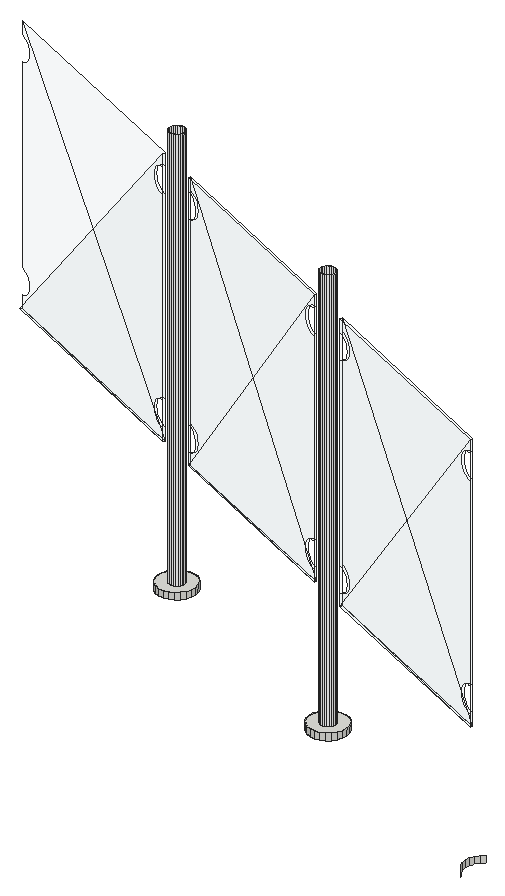
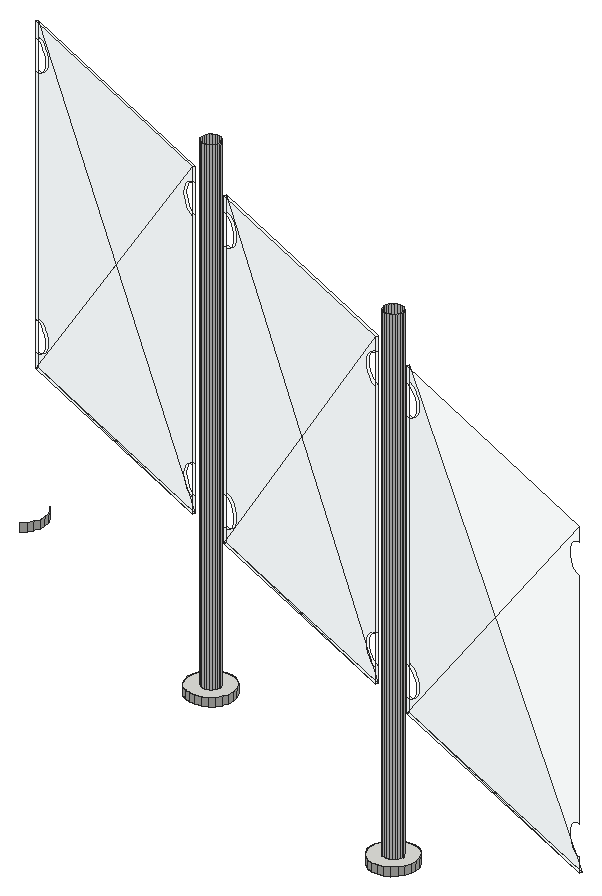
# SketchUp Ruby script. Lengths in inches.
U = 1.inch
M = Sketchup.active_model
def pt(a) = Geom::Point3d.new(a.map { |v| v * U })
def face(e, loops, mat)
  f = e.add_face(loops[0].map { |a| pt(a) })
  loops[1..].each { |l| e.add_face(l.map { |a| pt(a) }).erase! }
  f.material = f.back_material = mat if mat
  f
end
# faces: each face lists its corners as indices into pts; further lists are holes
def faces(e, pts, list, mat = nil) = list.each { |f| face(e, (f[0].is_a?(Array) ? f : [f]).map { |l| l.map { |i| pts[i] } }, mat) }
# xy, xz, yz: faces in a plane at the given z, y or x. An outline is a flat list of corners, or four numbers for a rectangle; further outlines are holes
def ring(l) = l.size == 4 ? [[l[0], l[1]], [l[2], l[1]], [l[2], l[3]], [l[0], l[3]]] : l.each_slice(2).to_a
def flat(e, list, mat, &to3) = list.each { |f| face(e, (f[0].is_a?(Array) ? f : [f]).map { |l| ring(l).map { |u, v| to3.(u, v) } }, mat) }
def xy(e, z, list, mat = nil) = flat(e, list, mat) { |x, y| [x, y, z] }
def xz(e, y, list, mat = nil) = flat(e, list, mat) { |x, z| [x, y, z] }
def yz(e, x, list, mat = nil) = flat(e, list, mat) { |y, z| [x, y, z] }
def lines(e, pts, list) = list.each { |a, b| e.add_line(pt(pts[a]), pt(pts[b])) }
# prism: a flat outline (further loops are holes) pulled along v
def prism(e, loops, v, mat = nil)
  f = face(e, loops, mat); d = Geom::Vector3d.new(v.map { |x| x * U })
  f.pushpull(f.normal.samedirection?(d) ? d.length : -d.length)
end
def box(e, o, s, mat = nil) = prism(e, [[o, [o[0] + s[0], o[1], o[2]], [o[0] + s[0], o[1] + s[1], o[2]], [o[0], o[1] + s[1], o[2]]]], [0, 0, s[2]], mat)
def at(x, y, z, deg = 0) = Geom::Transformation.translation(pt([x, y, z])) * Geom::Transformation.rotation(ORIGIN, Z_AXIS, deg.degrees)
def axes(o, x, y, z) = Geom::Transformation.new([*x, 0, *y, 0, *z, 0, *pt(o).to_a, 1])
def part(name) = M.definitions.add(name)
# library, detail: a bought-in or finely detailed component or shape, given as its bounding box
def library(name, o, s) = part(name).tap { |d| box(d.entities, o, s) }
def detail(e, o, s) = box(e.add_group.entities, o, s)
def put(e, d, t, mat = nil) = e.add_instance(d, t).tap { |i| i.material = mat if mat }
def group(e, t, mat = nil) = e.add_group.tap { |g| g.transformation = t; g.material = mat if mat }.entities
root = M.entities
M.materials.add("Glass_Safety_01").color = [204, 235, 244]
M.materials["Glass_Safety_01"].alpha = 0.1
M.materials.add("[Color_000]").color = [255, 255, 255]
xy(root,321.27,[[[766.1875,566.06,766.59,566.14,766.96,566.32,767.27,566.6,767.49,566.94,767.62,567.33,767.65,567.74,767.5625,568.14,767.38,568.51,767.11,568.82,766.76,569.04,766.375,569.17,765.96,569.2,765.5625,569.12,765.19,568.93,764.89,568.66,764.66,568.32,764.64,568.25,764.53,567.93,764.51,567.52,764.59,567.11,764.77,566.75,765.05,566.4375,765.39,566.21,765.78,566.08],[766.12,567,765.96,567.01,765.8,567.0625,765.66,567.15,765.55,567.28,765.48,567.42,765.45,567.58,765.46,567.75,765.5,567.88,765.51,567.9,765.6,568.04,765.72,568.15,765.87,568.22,766.03,568.26,766.2,568.25,766.35,568.19,766.49,568.1,766.6,567.98,766.67,567.83,766.7,567.67,766.69,567.51,766.65,567.38,766.64,567.35,766.55,567.22,766.43,567.11,766.28,567.03]],[767.51,567,767.62,567.33,767.65,567.74,767.5625,568.14,767.38,568.51,767.11,568.82,766.76,569.04,766.375,569.17,765.96,569.2,765.5625,569.12,765.19,568.93,764.89,568.66,764.66,568.32,764.64,568.25,765.5,567.88,765.51,567.9,765.6,568.04,765.72,568.15,765.87,568.22,766.03,568.26,766.2,568.25,766.35,568.19,766.49,568.1,766.6,567.98,766.67,567.83,766.7,567.67,766.69,567.51,766.65,567.38],[766.65,567.38,766.69,567.51,766.7,567.67,766.67,567.83,766.6,567.98,766.49,568.1,766.35,568.19,766.2,568.25,766.03,568.26,765.87,568.22,765.72,568.15,765.6,568.04,765.51,567.9,765.5,567.88],[[745.84,574.92,746.25,575,746.61,575.1875,746.92,575.46,747.15,575.8,747.28,576.19,747.3,576.6,747.22,577,747.03,577.37,746.76,577.68,746.42,577.91,746.03,578.04,745.62,578.06,745.21,577.98,744.85,577.79,744.54,577.52,744.3125,577.18,744.29,577.12,744.18,576.79,744.16,576.38,744.24,575.97,744.43,575.61,744.7,575.3,745.04,575.07,745.43,574.94],[745.78,575.86,745.61,575.87,745.45,575.92,745.32,576.01,745.21,576.14,745.13,576.28,745.1,576.44,745.11,576.61,745.16,576.74,745.16,576.76,745.25,576.9,745.375,577.01,745.52,577.08,745.68,577.12,745.85,577.11,746.01,577.06,746.14,576.97,746.25,576.84,746.33,576.7,746.36,576.53,746.35,576.37,746.3,576.24,746.3,576.21,746.21,576.08,746.08,575.97,745.9375,575.89]],[747.17,575.86,747.28,576.19,747.3,576.6,747.22,577,747.03,577.37,746.76,577.68,746.42,577.91,746.03,578.04,745.62,578.06,745.21,577.98,744.85,577.79,744.54,577.52,744.3125,577.18,744.29,577.12,745.16,576.74,745.16,576.76,745.25,576.9,745.375,577.01,745.52,577.08,745.68,577.12,745.85,577.11,746.01,577.06,746.14,576.97,746.25,576.84,746.33,576.7,746.36,576.53,746.35,576.37,746.3,576.24],
  [746.3,576.24,746.35,576.37,746.36,576.53,746.33,576.7,746.25,576.84,746.14,576.97,746.01,577.06,745.85,577.11,745.68,577.12,745.52,577.08,745.375,577.01,745.25,576.9,745.16,576.76,745.16,576.74]])
xy(root,321.27,[[766.12,567,766.28,567.03,766.43,567.11,766.55,567.22,766.64,567.35,766.65,567.38,765.5,567.88,765.46,567.75,765.45,567.58,765.48,567.42,765.55,567.28,765.66,567.15,765.8,567.0625,765.96,567.01],[745.78,575.86,745.9375,575.89,746.08,575.97,746.21,576.08,746.3,576.21,746.3,576.24,745.16,576.74,745.11,576.61,745.1,576.44,745.13,576.28,745.21,576.14,745.32,576.01,745.45,575.92,745.61,575.87]],"[Color_000]")
xy(root,321.86,[[766.1875,566.06,766.59,566.14,766.96,566.32,767.27,566.6,767.49,566.94,767.62,567.33,767.65,567.74,767.5625,568.14,767.38,568.51,767.11,568.82,766.76,569.04,766.375,569.17,765.96,569.2,765.5625,569.12,765.19,568.93,764.89,568.66,764.66,568.32,764.53,567.93,764.51,567.52,764.59,567.11,764.77,566.75,765.05,566.4375,765.39,566.21,765.78,566.08],[745.84,574.92,746.25,575,746.61,575.1875,746.92,575.46,747.15,575.8,747.28,576.19,747.3,576.6,747.22,577,747.03,577.37,746.76,577.68,746.42,577.91,746.03,578.04,745.62,578.06,745.21,577.98,744.85,577.79,744.54,577.52,744.3125,577.18,744.18,576.79,744.16,576.38,744.24,575.97,744.43,575.61,744.7,575.3,745.04,575.07,745.43,574.94]])
xy(root,331.9,[[785.36,559.12,767.84,566.75,767.92,566.93],[785.36,559.12,767.92,566.93,785.44,559.3],[764.39,568.25,747.5,575.61,747.57,575.79],[764.39,568.25,747.57,575.79,764.47,568.43],[744.03,577.12,724.79,585.5,724.87,585.68],
  [744.03,577.12,724.87,585.68,744.11,577.3]],"Glass_Safety_01")
p = [[785.75,557.61,321.27],[786.02,557.3,321.27],[786.02,557.3,321.86],[785.75,557.61,321.86],[785.5625,557.98,321.27],[785.5625,557.98,321.86],
  [785.48,558.38,321.27],[785.48,558.38,321.86],[785.51,558.79,321.27],[785.51,558.79,321.86],[785.64,559.18,321.27],[785.62,559.12,321.27],
  [785.64,559.18,321.86],[785.86,559.52,321.27],[785.86,559.52,321.86],[786.17,559.8,321.27],[786.17,559.8,321.86],[765.39,566.21,321.27],
  [765.78,566.08,321.27],[765.78,566.08,321.86],[765.39,566.21,321.86],[766.1875,566.06,321.27],[766.1875,566.06,321.86],[766.59,566.14,321.27],
  [766.59,566.14,321.86],[766.96,566.32,321.27],[766.96,566.32,321.86],[765.05,566.4375,321.27],[765.05,566.4375,321.86],[767.27,566.6,321.27],
  [767.27,566.6,321.86],[764.77,566.75,321.27],[764.77,566.75,321.86],[767.49,566.94,321.27],[767.49,566.94,321.86],[764.59,567.11,321.27],
  [764.59,567.11,321.86],[767.51,567,321.27],[767.62,567.33,321.27],[767.62,567.33,321.86],[765.8,567.0625,321.27],[765.96,567.01,321.27],
  [765.96,567.01,357.27],[765.8,567.0625,357.27],[766.12,567,321.27],[766.12,567,357.27],[766.28,567.03,321.27],[766.28,567.03,357.27],
  [766.43,567.11,321.27],[766.43,567.11,357.27],[764.51,567.52,321.27],[764.51,567.52,321.86],[765.66,567.15,321.27],[765.66,567.15,357.27],
  [766.55,567.22,321.27],[766.55,567.22,357.27],[765.55,567.28,321.27],[765.55,567.28,357.27],[766.64,567.35,321.27],[766.64,567.35,357.27],
  [765.48,567.42,321.27],[765.48,567.42,357.27],[767.65,567.74,321.27],[767.65,567.74,321.86],[765.45,567.58,321.27],[765.45,567.58,357.27],
  [766.65,567.38,321.27],[766.69,567.51,321.27],[766.69,567.51,357.27],[764.53,567.93,321.27],[764.53,567.93,321.86],[766.7,567.67,321.27],
  [766.7,567.67,357.27],[765.46,567.75,321.27],[765.46,567.75,357.27],[765.51,567.9,321.27],[765.5,567.88,321.27],[765.51,567.9,357.27],
  [766.67,567.83,321.27],[766.67,567.83,357.27],[767.5625,568.14,321.27],[767.5625,568.14,321.86],[766.6,567.98,321.27],[766.6,567.98,357.27],
  [764.66,568.32,321.27],[764.64,568.25,321.27],[764.66,568.32,321.86],[765.6,568.04,321.27],[765.6,568.04,357.27],[765.72,568.15,321.27],
  [765.72,568.15,357.27],[766.49,568.1,321.27],[766.49,568.1,357.27],[765.87,568.22,321.27],[765.87,568.22,357.27],[766.35,568.19,321.27],
  [766.35,568.19,357.27],[767.38,568.51,321.27],[767.38,568.51,321.86],[766.03,568.26,321.27],[766.03,568.26,357.27],[766.2,568.25,321.27],
  [766.2,568.25,357.27],[764.89,568.66,321.27],[764.89,568.66,321.86],[767.11,568.82,321.27],[767.11,568.82,321.86],[765.19,568.93,321.27],
  [765.19,568.93,321.86],[766.76,569.04,321.27],[766.76,569.04,321.86],[765.5625,569.12,321.27],[765.5625,569.12,321.86],[766.375,569.17,321.27],
  [766.375,569.17,321.86],[765.96,569.2,321.27],[765.96,569.2,321.86],[745.04,575.07,321.27],[745.43,574.94,321.27],[745.43,574.94,321.86],
  [745.04,575.07,321.86],[745.84,574.92,321.27],[745.84,574.92,321.86],[746.25,575,321.27],[746.25,575,321.86],[746.61,575.1875,321.27],
  [746.61,575.1875,321.86],[744.7,575.3,321.27],[744.7,575.3,321.86],[746.92,575.46,321.27],[746.92,575.46,321.86],[744.43,575.61,321.27],
  [744.43,575.61,321.86],[747.15,575.8,321.27],[747.15,575.8,321.86],[744.24,575.97,321.27],[744.24,575.97,321.86],[747.17,575.86,321.27],
  [747.28,576.19,321.27],[747.28,576.19,321.86],[745.32,576.01,321.27],[745.45,575.92,321.27],[745.45,575.92,357.27],[745.32,576.01,357.27],
  [745.61,575.87,321.27],[745.61,575.87,357.27],[745.78,575.86,321.27],[745.78,575.86,357.27],[745.9375,575.89,321.27],[745.9375,575.89,357.27],
  [746.08,575.97,321.27],[746.08,575.97,357.27],[744.16,576.38,321.27],[744.16,576.38,321.86],[745.21,576.14,321.27],[745.21,576.14,357.27],
  [746.21,576.08,321.27],[746.21,576.08,357.27],[745.13,576.28,321.27],[745.13,576.28,357.27],[746.3,576.21,321.27],[746.3,576.21,357.27],
  [746.3,576.24,321.27],[746.35,576.37,321.27],[746.35,576.37,357.27],[747.3,576.6,321.27],[747.3,576.6,321.86],[745.1,576.44,321.27],
  [745.1,576.44,357.27],[744.18,576.79,321.27],[744.18,576.79,321.86],[745.11,576.61,321.27],[745.11,576.61,357.27],[746.36,576.53,321.27],
  [746.36,576.53,357.27],[746.33,576.7,321.27],[746.33,576.7,357.27],[745.16,576.76,321.27],[745.16,576.74,321.27],[745.16,576.76,357.27],
  [747.22,577,321.27],[747.22,577,321.86],[746.25,576.84,321.27],[746.25,576.84,357.27],[744.3125,577.18,321.27],[744.29,577.12,321.27],
  [744.3125,577.18,321.86],[745.25,576.9,321.27],[745.25,576.9,357.27],[746.14,576.97,321.27],[746.14,576.97,357.27],[745.375,577.01,321.27],
  [745.375,577.01,357.27],[745.52,577.08,321.27],[745.52,577.08,357.27],[746.01,577.06,321.27],[746.01,577.06,357.27],[747.03,577.37,321.27],
  [747.03,577.37,321.86],[745.68,577.12,321.27],[745.68,577.12,357.27],[745.85,577.11,321.27],[745.85,577.11,357.27],[744.54,577.52,321.27],
  [744.54,577.52,321.86],[746.76,577.68,321.27],[746.76,577.68,321.86],[744.85,577.79,321.27],[744.85,577.79,321.86],[746.42,577.91,321.27],
  [746.42,577.91,321.86],[745.21,577.98,321.27],[745.21,577.98,321.86],[746.03,578.04,321.27],[746.03,578.04,321.86],[745.62,578.06,321.27],
  [745.62,578.06,321.86],[767.84,566.75,351.28],[767.84,566.75,335.125],[768.09,566.64,335.09],[768.33,566.54,334.98],[768.53,566.45,334.8125],
  [768.6875,566.38,334.59],[768.78,566.34,334.34],[768.82,566.33,334.0625],[768.78,566.34,333.79],[768.6875,566.38,333.53],[768.53,566.45,333.3125],
  [768.33,566.54,333.14],[768.09,566.64,333.04],[767.84,566.75,333],[767.84,566.75,331.9],[785.36,559.12,354.51],[767.84,566.75,354.51],
  [767.84,566.75,353.41],[768.09,566.64,353.37],[768.33,566.54,353.27],[768.53,566.45,353.1],[768.6875,566.38,352.88],[768.78,566.34,352.62],
  [768.82,566.33,352.35],[768.78,566.34,352.07],[768.6875,566.38,351.81],[768.53,566.45,351.59],[768.33,566.54,351.43],[768.09,566.64,351.32],
  [785.36,559.12,331.9],[785.36,559.12,333],[785.21,559.1875,333],[784.96,559.3,333.04],[784.72,559.4,333.14],[784.52,559.49,333.3125],
  [784.36,559.56,333.53],[784.27,559.6,333.79],[784.23,559.61,334.0625],[784.27,559.6,334.34],[784.36,559.56,334.59],[784.52,559.49,334.8125],
  [784.72,559.4,334.98],[784.96,559.3,335.09],[785.21,559.1875,335.125],[785.36,559.12,335.125],[785.36,559.12,351.28],[785.21,559.1875,351.28],
  [784.96,559.3,351.32],[784.72,559.4,351.43],[784.52,559.49,351.59],[784.36,559.56,351.81],[784.27,559.6,352.07],[784.23,559.61,352.35],
  [784.27,559.6,352.62],[784.36,559.56,352.88],[784.52,559.49,353.1],[784.72,559.4,353.27],[784.96,559.3,353.37],[785.21,559.1875,353.41],
  [785.36,559.12,353.41],[785.44,559.3,331.9],[785.44,559.3,333],[785.44,559.3,335.125],[785.44,559.3,351.28],[785.44,559.3,353.41],
  [785.44,559.3,354.51],[767.92,566.93,331.9],[767.92,566.93,333],[768.17,566.82,333.04],[768.41,566.72,333.14],[768.61,566.63,333.3125],
  [768.76,566.56,333.53],[768.86,566.52,333.79],[768.89,566.51,334.0625],[768.86,566.52,334.34],[768.76,566.56,334.59],[768.61,566.63,334.8125],
  [768.41,566.72,334.98],[768.17,566.82,335.09],[767.92,566.93,335.125],[767.92,566.93,351.28],[768.17,566.82,351.32],[768.41,566.72,351.43],
  [768.61,566.63,351.59],[768.76,566.56,351.81],[768.86,566.52,352.07],[768.89,566.51,352.35],[768.86,566.52,352.62],[768.76,566.56,352.88],
  [768.61,566.63,353.1],[768.41,566.72,353.27],[768.17,566.82,353.37],[767.92,566.93,353.41],[767.92,566.93,354.51],[785.29,559.37,335.125],
  [785.03,559.48,335.09],[784.8,559.58,334.98],[784.6,559.67,334.8125],[784.44,559.74,334.59],[784.35,559.78,334.34],[784.3125,559.79,334.0625],
  [784.35,559.78,333.79],[784.44,559.74,333.53],[784.6,559.67,333.3125],[784.8,559.58,333.14],[785.03,559.48,333.04],[785.29,559.37,333],
  [785.29,559.37,353.41],[785.03,559.48,353.37],[784.8,559.58,353.27],[784.6,559.67,353.1],[784.44,559.74,352.88],[784.35,559.78,352.62],
  [784.3125,559.79,352.35],[784.35,559.78,352.07],[784.44,559.74,351.81],[784.6,559.67,351.59],[784.8,559.58,351.43],[785.03,559.48,351.32],
  [785.29,559.37,351.28],[747.5,575.61,351.28],[747.5,575.61,335.125],[747.75,575.5,335.09],[747.98,575.4,334.98],[748.18,575.3125,334.8125],
  [748.34,575.25,334.59],[748.4375,575.2,334.34],[748.47,575.1875,334.0625],[748.4375,575.2,333.79],[748.34,575.25,333.53],[748.18,575.3125,333.3125],
  [747.98,575.4,333.14],[747.75,575.5,333.04],[747.5,575.61,333],[747.5,575.61,331.9],[764.39,568.25,354.51],[747.5,575.61,354.51],
  [747.5,575.61,353.41],[747.75,575.5,353.37],[747.98,575.4,353.27],[748.18,575.3125,353.1],[748.34,575.25,352.88],[748.4375,575.2,352.62],
  [748.47,575.1875,352.35],[748.4375,575.2,352.07],[748.34,575.25,351.81],[748.18,575.3125,351.59],[747.98,575.4,351.43],[747.75,575.5,351.32],
  [764.39,568.25,331.9],[764.39,568.25,333],[764.23,568.32,333],[763.98,568.43,333.04],[763.74,568.54,333.14],[763.54,568.625,333.3125],
  [763.39,568.69,333.53],[763.29,568.73,333.79],[763.26,568.75,334.0625],[763.29,568.73,334.34],[763.39,568.69,334.59],[763.54,568.625,334.8125],
  [763.74,568.54,334.98],[763.98,568.43,335.09],[764.23,568.32,335.125],[764.39,568.25,335.125],[764.39,568.25,351.28],[764.23,568.32,351.28],
  [763.98,568.43,351.32],[763.74,568.54,351.43],[763.54,568.625,351.59],[763.39,568.69,351.81],[763.29,568.73,352.07],[763.26,568.75,352.35],
  [763.29,568.73,352.62],[763.39,568.69,352.88],[763.54,568.625,353.1],[763.74,568.54,353.27],[763.98,568.43,353.37],[764.23,568.32,353.41],
  [764.39,568.25,353.41],[764.47,568.43,331.9],[764.47,568.43,333],[764.47,568.43,335.125],[764.47,568.43,351.28],[764.47,568.43,353.41],
  [764.47,568.43,354.51],[747.57,575.79,331.9],[747.57,575.79,333],[747.83,575.68,333.04],[748.0625,575.58,333.14],[748.26,575.49,333.3125],
  [748.42,575.43,333.53],[748.52,575.38,333.79],[748.55,575.37,334.0625],[748.52,575.38,334.34],[748.42,575.43,334.59],[748.26,575.49,334.8125],
  [748.0625,575.58,334.98],[747.83,575.68,335.09],[747.57,575.79,335.125],[747.57,575.79,351.28],[747.83,575.68,351.32],[748.0625,575.58,351.43],
  [748.26,575.49,351.59],[748.42,575.43,351.81],[748.52,575.38,352.07],[748.55,575.37,352.35],[748.52,575.38,352.62],[748.42,575.43,352.88],
  [748.26,575.49,353.1],[748.0625,575.58,353.27],[747.83,575.68,353.37],[747.57,575.79,353.41],[747.57,575.79,354.51],[764.3125,568.5,335.125],
  [764.06,568.61,335.09],[763.82,568.72,334.98],[763.62,568.8,334.8125],[763.47,568.87,334.59],[763.37,568.91,334.34],[763.34,568.93,334.0625],
  [763.37,568.91,333.79],[763.47,568.87,333.53],[763.62,568.8,333.3125],[763.82,568.72,333.14],[764.06,568.61,333.04],[764.3125,568.5,333],
  [764.3125,568.5,353.41],[764.06,568.61,353.37],[763.82,568.72,353.27],[763.62,568.8,353.1],[763.47,568.87,352.88],[763.37,568.91,352.62],
  [763.34,568.93,352.35],[763.37,568.91,352.07],[763.47,568.87,351.81],[763.62,568.8,351.59],[763.82,568.72,351.43],[764.06,568.61,351.32],
  [764.3125,568.5,351.28],[744.03,577.12,331.9],[744.03,577.12,333],[743.89,577.19,333],[743.63,577.3,333.04],[743.4,577.4,333.14],
  [743.2,577.49,333.3125],[743.04,577.55,333.53],[742.94,577.6,333.79],[742.91,577.61,334.0625],[742.94,577.6,334.34],[743.04,577.55,334.59],
  [743.2,577.49,334.8125],[743.4,577.4,334.98],[743.63,577.3,335.09],[743.89,577.19,335.125],[744.03,577.12,335.125],[744.03,577.12,351.28],
  [743.89,577.19,351.28],[743.63,577.3,351.32],[743.4,577.4,351.43],[743.2,577.49,351.59],[743.04,577.55,351.81],[742.94,577.6,352.07],
  [742.91,577.61,352.35],[742.94,577.6,352.62],[743.04,577.55,352.88],[743.2,577.49,353.1],[743.4,577.4,353.27],[743.63,577.3,353.37],
  [743.89,577.19,353.41],[744.03,577.12,353.41],[744.03,577.12,354.51],[724.79,585.5,331.9],[744.11,577.3,331.9],[744.11,577.3,333],
  [744.11,577.3,335.125],[744.11,577.3,351.28],[744.11,577.3,353.41],[744.11,577.3,354.51],[724.87,585.68,331.9],[724.87,585.68,333],
  [725.12,585.57,333.04],[725.36,585.47,333.14],[725.56,585.38,333.3125],[725.71,585.32,333.53],[725.81,585.27,333.79],[725.84,585.26,334.0625],
  [725.81,585.27,334.34],[725.71,585.32,334.59],[725.56,585.38,334.8125],[725.36,585.47,334.98],[725.12,585.57,335.09],[724.87,585.68,335.125],
  [724.87,585.68,351.28],[725.12,585.57,351.32],[725.36,585.47,351.43],[725.56,585.38,351.59],[725.71,585.32,351.81],[725.81,585.27,352.07],
  [725.84,585.26,352.35],[725.81,585.27,352.62],[725.71,585.32,352.88],[725.56,585.38,353.1],[725.36,585.47,353.27],[725.12,585.57,353.37],
  [724.87,585.68,353.41],[724.87,585.68,354.51],[743.96,577.37,335.125],[743.71,577.48,335.09],[743.48,577.58,334.98],[743.28,577.67,334.8125],
  [743.12,577.73,334.59],[743.02,577.78,334.34],[742.99,577.79,334.0625],[743.02,577.78,333.79],[743.12,577.73,333.53],[743.28,577.67,333.3125],
  [743.48,577.58,333.14],[743.71,577.48,333.04],[743.96,577.37,333],[743.96,577.37,353.41],[743.71,577.48,353.37],[743.48,577.58,353.27],
  [743.28,577.67,353.1],[743.12,577.73,352.88],[743.02,577.78,352.62],[742.99,577.79,352.35],[743.02,577.78,352.07],[743.12,577.73,351.81],
  [743.28,577.67,351.59],[743.48,577.58,351.43],[743.71,577.48,351.32],[743.96,577.37,351.28]]
faces(root,p,[[0,1,2,3],[4,0,3,5],[6,4,5,7],[8,6,7,9],[10,11,8,9,12],[13,10,12,14],[15,13,14,16],[17,18,19,20],
  [18,21,22,19],[21,23,24,22],[23,25,26,24],[27,17,20,28],[25,29,30,26],[31,27,28,32],[29,33,34,30],[35,31,32,36],
  [33,37,38,39,34],[50,35,36,51],[38,62,63,39],[69,50,51,70],[62,80,81,63],[84,85,69,70,86],[80,97,98,81],[103,84,86,104],
  [97,105,106,98],[107,103,104,108],[105,109,110,106],[111,107,108,112],[109,113,114,110],[115,111,112,116],[113,115,116,114],[117,118,119,120],
  [118,121,122,119],[121,123,124,122],[123,125,126,124],[127,117,120,128],[125,129,130,126],[131,127,128,132],[129,133,134,130],[135,131,132,136],
  [133,137,138,139,134],[152,135,136,153],[138,165,166,139],[169,152,153,170],[165,180,181,166],[184,185,169,170,186],[180,197,198,181],[203,184,186,204],
  [197,205,206,198],[207,203,204,208],[205,209,210,206],[211,207,208,212],[209,213,214,210],[215,211,212,216],[213,215,216,214]])
faces(root,p,[[40,41,42,43],[41,44,45,42],[44,46,47,45],[46,48,49,47],[52,40,43,53],[48,54,55,49],[56,52,53,57],[54,58,59,55],
  [60,56,57,61],[64,60,61,65],[58,66,67,68,59],[67,71,72,68],[73,64,65,74],[75,76,73,74,77],[71,78,79,72],[78,82,83,79],
  [87,75,77,88],[89,87,88,90],[82,91,92,83],[93,89,90,94],[91,95,96,92],[99,93,94,100],[101,99,100,102],[95,101,102,96],
  [140,141,142,143],[141,144,145,142],[144,146,147,145],[146,148,149,147],[148,150,151,149],[154,140,143,155],[150,156,157,151],[158,154,155,159],
  [156,160,161,157],[160,162,163,164,161],[167,158,159,168],[171,167,168,172],[163,173,174,164],[173,175,176,174],[177,178,171,172,179],[175,182,183,176],
  [187,177,179,188],[182,189,190,183],[191,187,188,192],[193,191,192,194],[189,195,196,190],[199,193,194,200],[201,199,200,202],[195,201,202,196]],"[Color_000]")
faces(root,p,[[217,218,219,220,221,222,223,224,225,226,227,228,229,230,231,232,233,234,235,236,237,238,239,240,241,242,243,244,245],[246,247,248,249,250,251,252,253,254,255,256,257,258,259,260,261,262,263,264,265,266,267,268,269,270,271,272,273,274,275,276,232,231],[246,277,278,279,280,281,282,232,276,262,261,247],[283,284,285,286,287,288,289,290,291,292,293,294,295,296,297,298,299,300,301,302,303,304,305,306,307,308,309,310,277],[280,279,311,312,313,314,315,316,317,318,319,320,321,322,323,278,277,310,282,281,324,325,326,327,328,329,330,331,332,333,334,335,336],[283,231,230,218,217,234,233,310,309,297,296,284],[337,338,339,340,341,342,343,344,345,346,347,348,349,350,351,352,353,354,355,356,357,358,359,360,361,362,363,364,365],[366,367,368,369,370,371,372,373,374,375,376,377,378,379,380,381,382,383,384,385,386,387,388,389,390,391,392,393,394,395,396,352,351],
  [366,397,398,399,400,401,402,352,396,382,381,367],[403,404,405,406,407,408,409,410,411,412,413,414,415,416,417,418,419,420,421,422,423,424,425,426,427,428,429,430,397],[400,399,431,432,433,434,435,436,437,438,439,440,441,442,443,398,397,430,402,401,444,445,446,447,448,449,450,451,452,453,454,455,456],[403,351,350,338,337,354,353,430,429,417,416,404],[457,458,459,460,461,462,463,464,465,466,467,468,469,470,471,472,473,474,475,476,477,478,479,480,481,482,483,484,485,486,487,488,489],[457,490,491,492,493,494,495,488,487,473,472,458],[496,497,498,499,500,501,502,503,504,505,506,507,508,509,510,511,512,513,514,515,516,517,518,519,520,521,522,523,490],[493,492,524,525,526,527,528,529,530,531,532,533,534,535,536,491,490,523,495,494,537,538,539,540,541,542,543,544,545,546,547,548,549]],"Glass_Safety_01")
